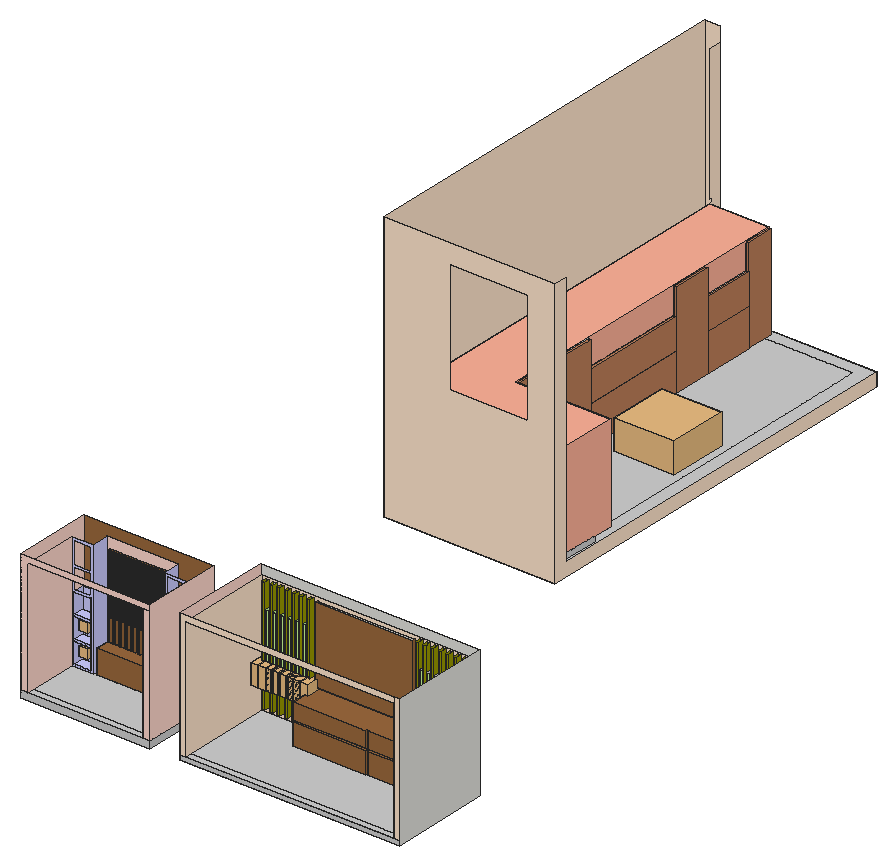
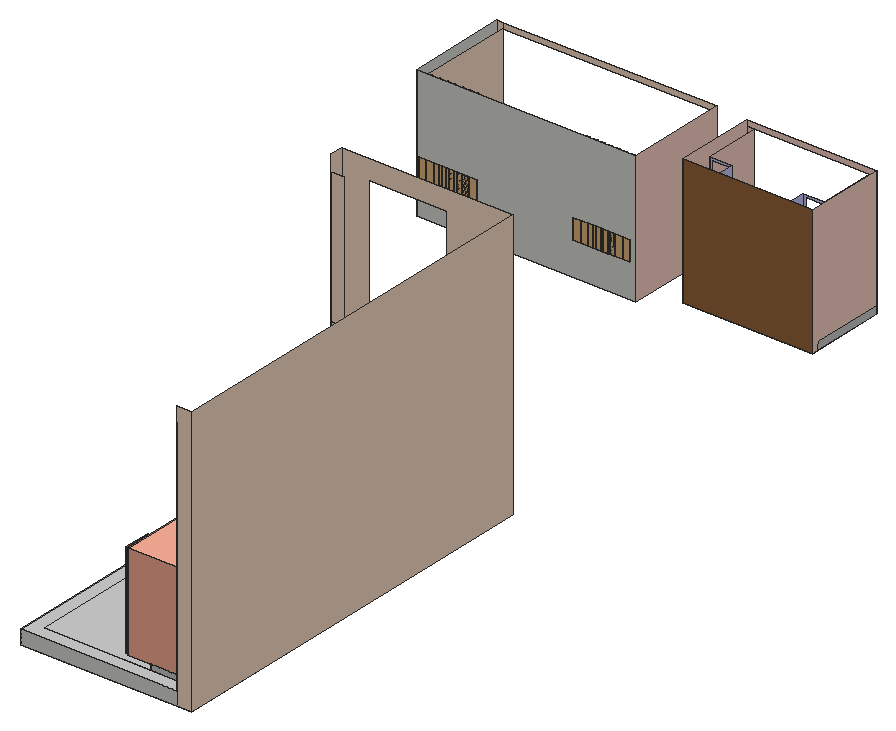
# SketchUp Ruby script. Lengths in inches.
U = 1.inch
M = Sketchup.active_model
def pt(a) = Geom::Point3d.new(a.map { |v| v * U })
def face(e, loops, mat)
  f = e.add_face(loops[0].map { |a| pt(a) })
  loops[1..].each { |l| e.add_face(l.map { |a| pt(a) }).erase! }
  f.material = f.back_material = mat if mat
  f
end
# faces: each face lists its corners as indices into pts; further lists are holes
def faces(e, pts, list, mat = nil) = list.each { |f| face(e, (f[0].is_a?(Array) ? f : [f]).map { |l| l.map { |i| pts[i] } }, mat) }
# xy, xz, yz: faces in a plane at the given z, y or x. An outline is a flat list of corners, or four numbers for a rectangle; further outlines are holes
def ring(l) = l.size == 4 ? [[l[0], l[1]], [l[2], l[1]], [l[2], l[3]], [l[0], l[3]]] : l.each_slice(2).to_a
def flat(e, list, mat, &to3) = list.each { |f| face(e, (f[0].is_a?(Array) ? f : [f]).map { |l| ring(l).map { |u, v| to3.(u, v) } }, mat) }
def xy(e, z, list, mat = nil) = flat(e, list, mat) { |x, y| [x, y, z] }
def xz(e, y, list, mat = nil) = flat(e, list, mat) { |x, z| [x, y, z] }
def yz(e, x, list, mat = nil) = flat(e, list, mat) { |y, z| [x, y, z] }
def lines(e, pts, list) = list.each { |a, b| e.add_line(pt(pts[a]), pt(pts[b])) }
# prism: a flat outline (further loops are holes) pulled along v
def prism(e, loops, v, mat = nil)
  f = face(e, loops, mat); d = Geom::Vector3d.new(v.map { |x| x * U })
  f.pushpull(f.normal.samedirection?(d) ? d.length : -d.length)
end
def box(e, o, s, mat = nil) = prism(e, [[o, [o[0] + s[0], o[1], o[2]], [o[0] + s[0], o[1] + s[1], o[2]], [o[0], o[1] + s[1], o[2]]]], [0, 0, s[2]], mat)
def at(x, y, z, deg = 0) = Geom::Transformation.translation(pt([x, y, z])) * Geom::Transformation.rotation(ORIGIN, Z_AXIS, deg.degrees)
def axes(o, x, y, z) = Geom::Transformation.new([*x, 0, *y, 0, *z, 0, *pt(o).to_a, 1])
def part(name) = M.definitions.add(name)
# library, detail: a bought-in or finely detailed component or shape, given as its bounding box
def library(name, o, s) = part(name).tap { |d| box(d.entities, o, s) }
def detail(e, o, s) = box(e.add_group.entities, o, s)
def put(e, d, t, mat = nil) = e.add_instance(d, t).tap { |i| i.material = mat if mat }
def group(e, t, mat = nil) = e.add_group.tap { |g| g.transformation = t; g.material = mat if mat }.entities
root = M.entities
M.materials.add("[Carrera Marble]").color = [207, 207, 207]
M.materials.add("[Color B01]").color = [255, 216, 204]
M.materials.add("[Color B02]").color = [255, 178, 153]
M.materials.add("[Color C01]").color = [255, 229, 204]
M.materials.add("[Color E07]").color = [153, 153, 0]
M.materials.add("[Color F02]").color = [204, 255, 153]
M.materials.add("[Color I01]").color = [204, 204, 255]
M.materials.add("[Wood Floor]").color = [155, 105, 61]
M.materials.add("[Wood Veneer 02]").color = [190, 128, 91]
c1 = library("Dome Light",[-12,-12,0],[24,24,12])
c2 = library("Spot Light\#1",[-5.1,-5.1,-11.05],[10.2,10.2,11.05])
c3 = library("Spot Light\#2",[-5.1,-5.1,-11.05],[10.2,10.2,11.05])
c4 = library("Omni Light",[-12,-12,-12],[24,24,24])
prism(root,[[[126.97,824.11,13.18],[126.78,870.57,13.18],[130.77,870.59,13.18],[130.95,824.12,13.18]]],[0,0,114.09],"[Wood Veneer 02]")
prism(root,[[[126.97,933.65,13.18],[126.59,966.6875,13.18],[130.19,966.73,13.18],[130.56,933.6875,13.18]]],[0,0,114.09],"[Wood Veneer 02]")
xy(root,-10.3125,[[38.18,499.97,244.12,983.1]])
xy(root,0,[[0,0,156.26,96.1875],[190.88,1.64,455.07,122.89]])
xy(root,5.5,[[197.89,1.64,448.06,8.66],[197.89,8.66,448.06,8.66,448.06,115.88,386.51,115.88,386.51,80.51,353.55,80.51,353.55,82.13,351.17,82.13,351.17,80.51,263.76,80.51,263.76,115.88,197.89,115.88]],"[Carrera Marble]")
xy(root,6.0625,[[228.71,515.38,244.12,515.38,244.12,983.1,55.53,983.1,55.53,967.6875,228.71,967.6875],[99.17,515.38,228.71,967.6875]],"[Carrera Marble]")
xy(root,8.6875,[[39.83,68.2,44.81,87.7],[47.15,68.2,52.13,84.32],[54.47,68.2,59.45,84.32],[61.79,68.2,66.77,84.32],[69.11,68.2,74.1,84.32],
  [76.43,68.2,81.42,84.32],[83.76,68.2,88.74,87.7],[91.08,68.2,96.06,84.32],[98.4,68.2,103.38,84.32],[105.72,68.2,110.7,87.7],
  [113.04,68.2,116.32,84.32],[47.15,84.32,52.13,87.7],[54.47,84.32,59.45,87.7],[61.79,84.32,66.77,87.7],[69.11,84.32,74.1,87.7],
  [76.43,84.32,81.42,87.7],[91.08,84.32,96.06,87.7],[98.4,84.32,103.38,87.7]])
xy(root,8.6875,[[8.49,0,147.15,8.49],[8.49,8.49,147.15,8.49,147.15,67.26,120.02,67.26,120.02,87.7,113.04,87.7,113.04,84.32,116.32,84.32,116.32,68.2,37.49,68.2,37.49,87.7,34.3,87.7,34.3,67.26,8.49,67.26]],"[Carrera Marble]")
xy(root,11.37,[[11.17,67.26,31.62,80.32]],"[Color I01]")
xy(root,11.4,[[122.73,67.26,144.4375,90.2]],"[Color I01]")
xy(root,11.5,[[202.89,109.94,206.54,115.88],[211.9,109.94,215.55,115.88],[215.55,109.94,215.57,115.88],[220.91,109.94,224.56,115.88],[229.92,109.94,233.57,115.88],
  [238.94,109.94,242.58,115.88],[247.95,109.94,251.59,115.88],[256.96,109.94,260.6,115.88],[388.06,109.94,391.7,115.88],[397.22,109.94,400.87,115.88],
  [406.39,109.94,410.03,115.88],[415.56,109.94,419.2,115.88],[419.2,109.94,419.22,115.88],[424.72,109.94,428.37,115.88],[433.89,109.94,437.53,115.88],
  [443.06,109.94,446.7,115.88]])
xy(root,12.375,[[55.53,515.38,55.53,967.6875,126.78,967.6875,126.78,823.17,131.14,823.17,131.14,696.23,126.78,696.23,126.78,586.56,241.2,586.56,241.2,515.38]])
xy(root,13.18,[[129.68,586.56,164.24,588.31],[164.74,586.56,240.3,588.31],[126.97,589.61,126.78,649.43,130.09,649.44,130.28,589.62],[126.97,650.36,126.78,695.33,130.09,695.35,130.28,650.375],[126.78,871.47,130.59,932.72]])
xy(root,31.1875,[[263.76,80.51,351.17,80.51,351.17,82.13,353.55,82.13,353.55,80.51,386.51,80.51,386.51,84.57,263.76,84.57]],"[Wood Floor]")
xy(root,33.9375,[[263.76,80.51,263.76,84.57,386.51,84.57,386.51,80.51,353.55,80.51,353.55,82.13,351.17,82.13,351.17,80.51]],"[Wood Floor]")
xy(root,36.07,[[11.17,67.26,31.62,80.32]],"[Color I01]")
xy(root,36.09,[[122.73,67.26,144.4375,90.2]])
xy(root,37.16,[[37.49,68.2,116.32,84.32]],"[Wood Floor]")
xy(root,38.07,[[11.17,67.26,31.62,80.32]],"[Color I01]")
xy(root,38.09,[[122.73,67.26,144.4375,90.2]],"[Color I01]")
xy(root,52.9375,[[263.76,80.51,351.17,80.51,351.17,82.13,353.55,82.13,353.55,80.51,386.51,80.51,386.51,115.88,263.76,115.88]],"[Wood Floor]")
xy(root,56.35,[[264.93,112.26,382.43,115.88]],"[Wood Floor]")
xy(root,58.06,[[126.78,696.23,131.14,823.17],[126.78,871.47,130.59,932.72]],"[Wood Veneer 02]")
xy(root,58.66,[[126.78,696.23,131.14,823.17],[115.09,871.47,126.28,932.72],[126.28,871.47,126.78,932.72],[126.78,871.47,130.59,932.72]])
xy(root,59.39,[[410.97,109.94,414.62,115.88]])
xy(root,59.66,[[243.44,109.94,247.09,115.88],[252.45,109.94,256.1,115.88],[392.64,109.94,396.28,115.88],[401.81,109.94,405.45,115.88]])
xy(root,60,[[420.14,109.94,423.78,115.88],[429.31,109.94,432.95,115.88]])
xy(root,60.5,[[207.4,109.94,211.04,115.88],[216.41,109.94,220.05,115.88],[225.42,109.94,229.06,115.88],[234.43,109.94,238.08,115.88]])
xy(root,60.52,[[438.47,109.94,442.12,115.88]])
xy(root,62.77,[[11.17,67.26,31.62,80.32]],"[Color I01]")
xy(root,62.78,[[122.73,67.26,144.4375,90.2]])
xy(root,64.25,[[41.15,84.32,43.49,87.7],[48.47,84.32,50.81,87.7],[55.79,84.32,58.13,87.7],[63.11,84.32,65.45,87.7],[70.43,84.32,72.77,87.7],
  [77.76,84.32,80.1,87.7],[85.08,84.32,87.42,87.7],[92.4,84.32,94.74,87.7],[99.72,84.32,102.06,87.7],[107.04,84.32,109.38,87.7],
  [114.36,84.32,116.7,87.7]])
xy(root,64.77,[[11.17,67.26,31.62,80.32]],"[Color I01]")
xy(root,64.78,[[122.73,67.26,144.4375,90.2]],"[Color I01]")
xy(root,80.6,[[164.74,586.56,240.3,588.31]],"[Wood Veneer 02]")
xy(root,95.53,[[115.09,871.47,126.28,932.72],[126.28,871.47,126.78,932.72]])
xy(root,95.53,[[126.78,696.23,131.14,823.17],[126.78,871.47,130.59,932.72]],"[Wood Veneer 02]")
xy(root,127.26,[[129.68,586.56,164.24,588.31],[126.97,589.61,130.28,589.62,130.09,649.44,126.78,649.43],[126.97,650.36,130.28,650.375,130.09,695.35,126.78,695.33]],"[Wood Veneer 02]")
xz(root,0,[[0,0,156.26,8.6875]],"[Carrera Marble]")
xz(root,0,[[0,8.6875,8.49,8.6875,8.49,148.5,156.26,148.5,156.26,155.125,0,155.125],[147.15,8.6875,156.26,148.5]],"[Color B01]")
xz(root,1.64,[[190.88,0,455.07,5.5]],"[Carrera Marble]")
xz(root,1.64,[[190.88,5.5,197.89,5.5,197.89,151.1875,448.06,151.1875,448.06,158,190.88,158],[448.06,5.5,455.07,158]],"[Color C01]")
xz(root,67.26,[[[8.49,8.6875,34.3,147.5625],[11.17,118.18,31.62,144.88],[11.17,64.77,31.62,89.48],[11.17,11.37,31.62,36.07],[11.17,38.07,31.62,62.77],[11.17,91.48,31.62,116.18]],[[120.02,8.6875,147.15,147.5625],[122.73,118.16,144.4375,144.85],[122.73,64.78,144.4375,89.47],[122.73,38.09,144.4375,62.78],[122.73,11.4,144.4375,36.09],[122.73,91.47,144.4375,116.16]]],"[Color I01]")
xz(root,68.2,[[37.49,8.6875,116.32,37.16]],"[Wood Floor]")
xz(root,80.32,[[11.17,11.37,31.62,36.07],[11.17,38.07,31.62,62.77],[11.17,64.77,31.62,89.48]],"[Color I01]")
xz(root,80.51,[[263.76,5.5,351.17,31.1875],[353.55,5.5,386.51,31.1875],[263.76,33.9375,351.17,52.9375],[353.55,33.9375,386.51,52.9375]],"[Wood Floor]")
xz(root,82.13,[[351.17,5.5,353.55,31.1875],[351.17,33.9375,353.55,52.9375]],"[Wood Floor]")
xz(root,84.32,[[37.49,8.6875,52.13,37.16],[52.13,8.6875,59.45,37.16],[59.45,8.6875,66.77,37.16],[66.77,8.6875,74.1,37.16],[74.1,8.6875,81.42,37.16],
  [81.42,8.6875,96.06,37.16],[96.06,8.6875,103.38,37.16],[103.38,8.6875,110.7,37.16],[110.7,8.6875,116.32,37.16]])
xz(root,84.57,[[263.76,31.1875,386.51,33.9375]],"[Wood Floor]")
xz(root,87.7,[[[34.3,8.6875,37.49,8.6875,37.49,135.5625,39.83,135.5625,39.83,8.6875,44.81,8.6875,44.81,135.5625,47.15,135.5625,47.15,8.6875,52.13,8.6875,52.13,135.5625,54.47,135.5625,54.47,8.6875,59.45,8.6875,59.45,135.5625,61.79,135.5625,61.79,8.6875,66.77,8.6875,66.77,135.5625,69.11,135.5625,69.11,8.6875,74.1,8.6875,74.1,135.5625,76.43,135.5625,76.43,8.6875,81.42,8.6875,81.42,135.5625,83.76,135.5625,83.76,8.6875,88.74,8.6875,88.74,135.5625,91.08,135.5625,91.08,8.6875,96.06,8.6875,96.06,135.5625,98.4,135.5625,98.4,8.6875,103.38,8.6875,103.38,135.5625,105.72,135.5625,105.72,8.6875,110.7,8.6875,110.7,135.5625,113.04,135.5625,113.04,8.6875,120.02,8.6875,120.02,148.5,34.3,148.5],[41.15,64.25,43.49,135.5625],[48.47,64.25,50.81,135.5625],[55.79,64.25,58.13,135.5625],[63.11,64.25,65.45,135.5625],[70.43,64.25,72.77,135.5625],[77.76,64.25,80.1,135.5625],[85.08,64.25,87.42,135.5625],[92.4,64.25,94.74,135.5625],[99.72,64.25,102.06,135.5625],[107.04,64.25,109.38,135.5625],[114.36,64.25,116.7,135.5625]]],"[Color B01]")
xz(root,90.2,[[122.73,11.4,144.4375,36.09],[122.73,38.09,144.4375,62.78],[122.73,64.78,144.4375,89.47]],"[Color I01]")
xz(root,96.1875,[[0,0,156.26,155.125]],"[Wood Floor]")
xz(root,109.94,[[202.89,11.5,206.54,149],[211.9,11.5,215.55,149],[220.91,11.5,224.56,149],[229.92,11.5,233.57,149],[238.94,11.5,242.58,149],
  [247.95,11.5,251.59,149],[256.96,11.5,260.6,149],[388.06,11.5,391.7,149],[397.22,11.5,400.87,149],[406.39,11.5,410.03,149],
  [415.56,11.5,419.2,149],[424.72,11.5,428.37,149],[433.89,11.5,437.53,149],[443.06,11.5,446.7,149]],"[Color E07]")
xz(root,109.94,[[410.97,59.39,414.62,120.1875],[243.44,59.66,247.09,120.1875],[252.45,59.66,256.1,120.1875],[392.64,59.66,396.28,120.1875],[401.81,59.66,405.45,120.1875],
  [420.14,60,423.78,120.1875],[429.31,60,432.95,120.1875],[207.4,60.5,211.04,120.1875],[216.41,60.5,220.05,120.1875],[225.42,60.5,229.06,120.1875],
  [234.43,60.5,238.08,120.1875],[438.47,60.52,442.12,120.1875]],"[Color F02]")
xz(root,112.26,[[264.93,56.35,382.43,147.04]],"[Wood Floor]")
xz(root,115.88,[[211.9,11.5,215.55,149],[220.91,11.5,224.56,149],[229.92,11.5,233.57,149],[238.94,11.5,242.58,149],[247.95,11.5,251.59,149],
  [256.96,11.5,260.6,149],[388.06,11.5,391.7,149],[397.22,11.5,400.87,149],[406.39,11.5,410.03,149],[415.56,11.5,419.2,149],
  [424.72,11.5,428.37,149],[433.89,11.5,437.53,149],[443.06,11.5,446.7,149],[410.97,59.39,414.62,120.1875],[243.44,59.66,247.09,120.1875],
  [252.45,59.66,256.1,120.1875],[392.64,59.66,396.28,120.1875],[401.81,59.66,405.45,120.1875],[420.14,60,423.78,120.1875],[429.31,60,432.95,120.1875],
  [207.4,60.5,211.04,120.1875],[216.41,60.5,220.05,120.1875],[225.42,60.5,229.06,120.1875],[234.43,60.5,238.08,120.1875],[438.47,60.52,442.12,120.1875]])
xz(root,115.88,[[[197.89,5.5,263.76,5.5,263.76,52.9375,386.51,52.9375,386.51,5.5,448.06,5.5,448.06,151.1875,197.89,151.1875],[264.93,56.35,382.43,147.04],[202.89,11.5,206.54,149],[211.9,11.5,215.55,149],[220.91,11.5,224.56,149],[229.92,11.5,233.57,149],[238.94,11.5,242.58,149],[247.95,11.5,251.59,149],[256.96,11.5,260.6,149],[388.06,11.5,391.7,149],[397.22,11.5,400.87,149],[406.39,11.5,410.03,149],[415.56,11.5,419.2,149],[424.72,11.5,428.37,149],[433.89,11.5,437.53,149],[443.06,11.5,446.7,149],[410.97,59.39,414.62,120.1875],[243.44,59.66,247.09,120.1875],[252.45,59.66,256.1,120.1875],[401.81,59.66,405.45,120.1875],[392.64,59.66,396.28,120.1875],[420.14,60,423.78,120.1875],[429.31,60,432.95,120.1875],[207.4,60.5,211.04,120.1875],[216.41,60.5,220.05,120.1875],[225.42,60.5,229.06,120.1875],[234.43,60.5,238.08,120.1875],[438.47,60.52,442.12,120.1875]]],"[Color C01]")
xz(root,122.89,[[190.88,0,455.07,158]])
xz(root,499.97,[[[38.18,-10.3125,244.12,313],[116.72,153.625,211.22,289.75]]],"[Color C01]")
xz(root,515.38,[[99.17,6.0625,228.71,12.375],[55.53,12.375,99.17,132.5625],[99.17,12.375,228.71,132.5625],[228.71,12.375,228.71,132.5625,243.82,132.5625,243.82,128.0625,241.2,128.0625,241.2,12.375]])
xz(root,515.38,[[228.71,6.0625,228.71,12.375,241.2,12.375,241.2,128.0625,243.82,128.0625,243.82,132.5625,228.71,132.5625,228.71,294.5,244.12,294.5,244.12,6.0625]],"[Color C01]")
xz(root,586.56,[[129.68,13.18,164.24,127.26],[164.74,13.18,240.3,80.6]])
xz(root,588.31,[[129.68,13.18,164.24,127.26],[164.74,13.18,240.3,80.6]],"[Wood Veneer 02]")
xz(root,696.23,[[126.78,12.375,131.14,58.06],[126.78,58.66,131.14,95.53]],"[Wood Veneer 02]")
xz(root,823.17,[[126.78,12.375,131.14,58.06],[126.78,58.66,131.14,95.53]],"[Color B02]")
xz(root,871.47,[[115.09,58.66,126.28,95.53],[126.28,58.66,126.78,95.53]])
xz(root,871.47,[[126.78,13.18,130.59,58.06],[126.78,58.66,130.59,95.53]],"[Wood Veneer 02]")
xz(root,932.72,[[115.09,58.66,126.28,95.53],[126.28,58.66,126.78,95.53]])
xz(root,932.72,[[126.78,13.18,130.59,58.06]],"[Color B02]")
xz(root,932.72,[[126.78,58.66,130.59,95.53]],"[Wood Veneer 02]")
xz(root,983.1,[[55.53,-10.3125,244.12,6.0625]])
xz(root,983.1,[[38.18,-10.3125,55.53,313]],"[Color C01]")
yz(root,0,[[0,0,87.7,8.6875]],"[Carrera Marble]")
yz(root,0,[[87.7,0,87.7,8.6875,0,8.6875,0,155.125,96.1875,155.125,96.1875,0]],"[Color B01]")
yz(root,8.49,[[0,8.6875,67.26,147.5625]],"[Color B01]")
yz(root,11.17,[[67.26,11.37,80.32,36.07],[67.26,38.07,80.32,62.77],[67.26,64.77,80.32,89.48]],"[Color I01]")
yz(root,31.62,[[67.26,36.07,80.32,38.07],[67.26,62.77,80.32,64.77]])
yz(root,31.62,[[67.26,11.37,80.32,36.07],[67.26,38.07,80.32,62.77],[67.26,64.77,80.32,89.48]],"[Color I01]")
yz(root,34.3,[[67.26,8.6875,87.7,147.5625]],"[Color I01]")
yz(root,37.49,[[68.2,8.6875,84.32,37.16]],"[Wood Floor]")
yz(root,38.18,[[499.97,-10.3125,983.1,313]],"[Color C01]")
yz(root,48.47,[[84.32,64.25,87.7,135.5625]],"[Wood Floor]")
yz(root,52.13,[[84.32,8.6875,87.7,135.5625]],"[Wood Floor]")
yz(root,55.53,[[515.38,12.375,967.6875,128.0625]])
yz(root,55.53,[[967.6875,6.0625,983.1,6.0625,983.1,294.5,967.6875,294.5,967.6875,132.5625,971,132.5625,971,128.0625,967.6875,128.0625]],"[Color C01]")
yz(root,55.79,[[84.32,64.25,87.7,135.5625]],"[Wood Floor]")
yz(root,59.45,[[84.32,8.6875,87.7,135.5625]],"[Wood Floor]")
yz(root,63.11,[[84.32,64.25,87.7,135.5625]],"[Wood Floor]")
yz(root,66.77,[[84.32,8.6875,87.7,135.5625]],"[Wood Floor]")
yz(root,70.43,[[84.32,64.25,87.7,135.5625]],"[Wood Floor]")
yz(root,74.1,[[84.32,8.6875,87.7,135.5625]],"[Wood Floor]")
yz(root,77.76,[[84.32,64.25,87.7,135.5625]],"[Wood Floor]")
yz(root,81.42,[[84.32,8.6875,87.7,135.5625]],"[Wood Floor]")
yz(root,85.08,[[84.32,64.25,87.7,135.5625]],"[Wood Floor]")
yz(root,92.4,[[84.32,64.25,87.7,135.5625]],"[Wood Floor]")
yz(root,96.06,[[84.32,8.6875,87.7,135.5625]],"[Wood Floor]")
yz(root,99.72,[[84.32,64.25,87.7,135.5625]],"[Wood Floor]")
yz(root,103.38,[[84.32,8.6875,87.7,135.5625]],"[Wood Floor]")
yz(root,107.04,[[84.32,64.25,87.7,135.5625]],"[Wood Floor]")
yz(root,110.7,[[84.32,8.6875,87.7,135.5625]],"[Wood Floor]")
yz(root,114.36,[[84.32,64.25,87.7,135.5625]],"[Wood Floor]")
yz(root,115.09,[[871.47,58.66,932.72,95.53]])
yz(root,116.32,[[68.2,8.6875,84.32,37.16]],"[Wood Floor]")
yz(root,120.02,[[67.26,8.6875,87.7,147.5625]],"[Color I01]")
yz(root,122.73,[[67.26,11.4,90.2,36.09],[67.26,38.09,90.2,62.78],[67.26,64.78,90.2,89.47]],"[Color I01]")
yz(root,126.28,[[871.47,58.66,932.72,95.53]])
yz(root,126.78,[[871.47,13.18,932.72,58.06],[696.23,58.66,823.17,95.53],[871.47,58.66,932.72,95.53]])
yz(root,129.68,[[586.56,13.18,588.31,127.26]])
yz(root,130.59,[[871.47,13.18,932.72,58.06],[871.47,58.66,932.72,95.53]],"[Wood Veneer 02]")
yz(root,131.14,[[696.23,12.375,823.17,58.06],[696.23,58.66,823.17,95.53]],"[Wood Veneer 02]")
yz(root,144.4375,[[67.26,36.09,90.2,38.09],[67.26,62.78,90.2,64.78]])
yz(root,144.4375,[[67.26,11.4,90.2,36.09],[67.26,38.09,90.2,62.78],[67.26,64.78,90.2,89.47]],"[Color I01]")
yz(root,147.15,[[0,8.6875,67.26,147.5625]],"[Color B01]")
yz(root,156.26,[[0,0,87.7,8.6875]],"[Carrera Marble]")
yz(root,156.26,[[87.7,0,96.1875,0,96.1875,155.125,0,155.125,0,8.6875,87.7,8.6875]],"[Color B01]")
yz(root,164.24,[[586.56,13.18,588.31,127.26]],"[Color B02]")
yz(root,164.74,[[586.56,13.18,588.31,80.6]])
yz(root,190.88,[[1.64,0,122.89,158]],"[Color B01]")
yz(root,197.89,[[1.64,5.5,115.88,151.1875]],"[Color C01]")
yz(root,202.89,[[109.94,11.5,115.88,149]],"[Color E07]")
yz(root,206.54,[[109.94,11.5,115.88,149]],"[Color E07]")
yz(root,207.4,[[109.94,60.5,115.88,120.1875]],"[Color F02]")
yz(root,211.04,[[109.94,60.5,115.88,120.1875]],"[Color F02]")
yz(root,211.9,[[109.94,11.5,115.88,149]],"[Color E07]")
yz(root,215.55,[[109.94,11.5,115.88,149]],"[Color E07]")
yz(root,216.41,[[109.94,60.5,115.88,120.1875]],"[Color F02]")
yz(root,220.05,[[109.94,60.5,115.88,120.1875]],"[Color F02]")
yz(root,220.91,[[109.94,11.5,115.88,149]],"[Color E07]")
yz(root,224.56,[[109.94,11.5,115.88,149]],"[Color E07]")
yz(root,225.42,[[109.94,60.5,115.88,120.1875]],"[Color F02]")
yz(root,229.06,[[109.94,60.5,115.88,120.1875]],"[Color F02]")
yz(root,229.92,[[109.94,11.5,115.88,149]],"[Color E07]")
yz(root,233.57,[[109.94,11.5,115.88,149]],"[Color E07]")
yz(root,234.43,[[109.94,60.5,115.88,120.1875]],"[Color F02]")
yz(root,238.08,[[109.94,60.5,115.88,120.1875]],"[Color F02]")
yz(root,238.94,[[109.94,11.5,115.88,149]],"[Color E07]")
yz(root,240.3,[[586.56,13.18,588.31,80.6]],"[Wood Veneer 02]")
yz(root,242.58,[[109.94,11.5,115.88,149]],"[Color E07]")
yz(root,243.44,[[109.94,59.66,115.88,120.1875]],"[Color F02]")
yz(root,244.12,[[499.97,-10.3125,983.1,-10.3125,983.1,6.0625,515.38,6.0625,515.38,313,499.97,313]],"[Color C01]")
yz(root,247.09,[[109.94,59.66,115.88,120.1875]])
yz(root,247.95,[[109.94,11.5,115.88,149]],"[Color E07]")
yz(root,251.59,[[109.94,11.5,115.88,149]],"[Color E07]")
yz(root,252.45,[[109.94,59.66,115.88,120.1875]],"[Color F02]")
yz(root,256.1,[[109.94,59.66,115.88,120.1875]],"[Color F02]")
yz(root,256.96,[[109.94,11.5,115.88,149]],"[Color E07]")
yz(root,260.6,[[109.94,11.5,115.88,149]],"[Color E07]")
yz(root,263.76,[[80.51,5.5,80.51,31.1875,84.57,31.1875,84.57,33.9375,80.51,33.9375,80.51,52.9375,115.88,52.9375,115.88,5.5]],"[Wood Floor]")
yz(root,264.93,[[112.26,56.35,115.88,147.04]],"[Wood Floor]")
yz(root,351.17,[[80.51,5.5,82.13,31.1875],[80.51,33.9375,82.13,52.9375]],"[Wood Floor]")
yz(root,353.55,[[80.51,5.5,82.13,31.1875],[80.51,33.9375,82.13,52.9375]],"[Wood Floor]")
yz(root,382.43,[[112.26,56.35,115.88,147.04]],"[Wood Floor]")
yz(root,386.51,[[80.51,5.5,115.88,5.5,115.88,52.9375,80.51,52.9375,80.51,33.9375,84.57,33.9375,84.57,31.1875,80.51,31.1875]],"[Wood Floor]")
yz(root,388.06,[[109.94,11.5,115.88,149]],"[Color E07]")
yz(root,391.7,[[109.94,11.5,115.88,149]],"[Color E07]")
yz(root,392.64,[[109.94,59.66,115.88,120.1875]])
yz(root,396.28,[[109.94,59.66,115.88,120.1875]],"[Color F02]")
yz(root,397.22,[[109.94,11.5,115.88,149]],"[Color E07]")
yz(root,400.87,[[109.94,11.5,115.88,149]],"[Color E07]")
yz(root,401.81,[[109.94,59.66,115.88,120.1875]])
yz(root,405.45,[[109.94,59.66,115.88,120.1875]],"[Color F02]")
yz(root,406.39,[[109.94,11.5,115.88,149]],"[Color E07]")
yz(root,410.03,[[109.94,11.5,115.88,149]],"[Color E07]")
yz(root,410.97,[[109.94,59.39,115.88,120.1875]])
yz(root,414.62,[[109.94,59.39,115.88,120.1875]],"[Color F02]")
yz(root,415.56,[[109.94,11.5,115.88,149]],"[Color E07]")
yz(root,419.2,[[109.94,11.5,115.88,149]],"[Color E07]")
yz(root,420.14,[[109.94,60,115.88,120.1875]])
yz(root,423.78,[[109.94,60,115.88,120.1875]],"[Color F02]")
yz(root,424.72,[[109.94,11.5,115.88,149]],"[Color E07]")
yz(root,428.37,[[109.94,11.5,115.88,149]],"[Color E07]")
yz(root,429.31,[[109.94,60,115.88,120.1875]])
yz(root,432.95,[[109.94,60,115.88,120.1875]],"[Color F02]")
yz(root,433.89,[[109.94,11.5,115.88,149]],"[Color E07]")
yz(root,437.53,[[109.94,11.5,115.88,149]],"[Color E07]")
yz(root,438.47,[[109.94,60.52,115.88,120.1875]])
yz(root,442.12,[[109.94,60.52,115.88,120.1875]],"[Color F02]")
yz(root,443.06,[[109.94,11.5,115.88,149]],"[Color E07]")
yz(root,446.7,[[109.94,11.5,115.88,149]],"[Color E07]")
yz(root,448.06,[[1.64,5.5,115.88,151.1875]],"[Color C01]")
yz(root,455.07,[[1.64,0,122.89,158]])
p = [[126.97,589.61,13.18],[126.97,589.61,127.26],[126.78,649.43,127.26],[126.78,649.43,13.18],[130.28,589.62,13.18],[130.28,589.62,127.26],
  [130.09,649.44,13.18],[130.09,649.44,127.26],[126.78,695.33,127.26],[126.78,695.33,13.18],[126.97,650.36,13.18],[126.97,650.36,127.26],
  [130.28,650.375,13.18],[130.28,650.375,127.26],[130.09,695.35,13.18],[130.09,695.35,127.26]]
faces(root,p,[[0,1,2,3],[1,0,4,5],[8,9,10,11]])
faces(root,p,[[5,4,6,7],[3,2,7,6],[11,10,12,13],[14,15,13,12]],"[Wood Veneer 02]")
faces(root,p,[[9,8,15,14]],"[Color B02]")
put(root,c1,axes([182.73,745.84,6.0625],[3,0,0],[0,3,0],[0,0,3]),"[Color I01]")
g1 = group(root,at(55.53,515.38,6.0625),"[Carrera Marble]")
xy(g1,0,[[43.64,0,185.67,48.25]])
xy(g1,6.3125,[[0,0,185.67,0,185.67,48.25,43.64,48.25,43.64,452.31,0,452.31]],"[Carrera Marble]")
xz(g1,0,[[43.64,0,185.67,6.3125]])
xz(g1,48.25,[[43.64,0,185.67,6.3125]],"[Carrera Marble]")
xz(g1,452.31,[[0,0,43.64,6.3125]])
yz(g1,43.64,[[48.25,0,452.31,6.3125]])
yz(g1,185.67,[[0,0,48.25,6.3125]],"[Carrera Marble]")
g2 = group(root,at(37.49,84.32,8.6875),"[Wood Floor]")
xy(g2,126.875,[[0,0,2.34,3.375],[3.66,0,6,3.375],[7.32,0,9.66,3.375],[10.98,0,13.32,3.375],[14.64,0,16.98,3.375],
  [18.3,0,20.64,3.375],[21.96,0,24.3,3.375],[25.625,0,27.96,3.375],[29.29,0,31.625,3.375],[32.95,0,35.29,3.375],
  [36.61,0,38.95,3.375],[40.27,0,42.61,3.375],[43.93,0,46.27,3.375],[47.59,0,49.93,3.375],[51.25,0,53.59,3.375],
  [54.91,0,57.25,3.375],[58.57,0,60.91,3.375],[62.23,0,64.57,3.375],[65.89,0,68.23,3.375],[69.55,0,71.89,3.375],
  [73.21,0,75.55,3.375],[76.875,0,79.21,3.375]],"[Wood Floor]")
xz(g2,0,[[0,0,2.34,126.875],[7.32,0,9.66,126.875],[14.64,0,16.98,126.875],[21.96,0,24.3,126.875],[29.29,0,31.625,126.875],
  [36.61,0,38.95,126.875],[43.93,0,46.27,126.875],[51.25,0,53.59,126.875],[58.57,0,60.91,126.875],[65.89,0,68.23,126.875],
  [73.21,0,75.55,126.875],[3.66,55.5625,6,126.875],[10.98,55.5625,13.32,126.875],[18.3,55.5625,20.64,126.875],[25.625,55.5625,27.96,126.875],
  [32.95,55.5625,35.29,126.875],[40.27,55.5625,42.61,126.875],[47.59,55.5625,49.93,126.875],[54.91,55.5625,57.25,126.875],[62.23,55.5625,64.57,126.875],
  [69.55,55.5625,71.89,126.875],[76.875,55.5625,79.21,126.875]],"[Wood Floor]")
yz(g2,0,[[0,0,3.375,126.875]],"[Wood Floor]")
yz(g2,2.34,[[0,0,3.375,126.875]],"[Wood Floor]")
yz(g2,3.66,[[0,55.5625,3.375,126.875]],"[Wood Floor]")
yz(g2,6,[[0,55.5625,3.375,126.875]],"[Wood Floor]")
yz(g2,7.32,[[0,0,3.375,126.875]],"[Wood Floor]")
yz(g2,9.66,[[0,0,3.375,126.875]],"[Wood Floor]")
yz(g2,13.32,[[0,55.5625,3.375,126.875]])
yz(g2,16.98,[[0,0,3.375,126.875]],"[Wood Floor]")
yz(g2,20.64,[[0,55.5625,3.375,126.875]],"[Wood Floor]")
yz(g2,24.3,[[0,0,3.375,126.875]],"[Wood Floor]")
yz(g2,27.96,[[0,55.5625,3.375,126.875]],"[Wood Floor]")
yz(g2,31.625,[[0,0,3.375,126.875]],"[Wood Floor]")
yz(g2,35.29,[[0,55.5625,3.375,126.875]],"[Wood Floor]")
yz(g2,38.95,[[0,0,3.375,126.875]],"[Wood Floor]")
yz(g2,42.61,[[0,55.5625,3.375,126.875]],"[Wood Floor]")
yz(g2,46.27,[[0,0,3.375,126.875]],"[Wood Floor]")
yz(g2,49.93,[[0,55.5625,3.375,126.875]],"[Wood Floor]")
yz(g2,51.25,[[0,0,3.375,126.875]])
yz(g2,53.59,[[0,0,3.375,126.875]],"[Wood Floor]")
yz(g2,57.25,[[0,55.5625,3.375,126.875]],"[Wood Floor]")
yz(g2,60.91,[[0,0,3.375,126.875]],"[Wood Floor]")
yz(g2,64.57,[[0,55.5625,3.375,126.875]],"[Wood Floor]")
yz(g2,68.23,[[0,0,3.375,126.875]],"[Wood Floor]")
yz(g2,71.89,[[0,55.5625,3.375,126.875]],"[Wood Floor]")
yz(g2,75.55,[[0,0,3.375,126.875]],"[Wood Floor]")
yz(g2,79.21,[[0,55.5625,3.375,126.875]],"[Wood Floor]")
g3 = group(root,at(55.53,515.38,12.375),"[Color B02]")
xy(g3,115.6875,[[0,0,185.67,0,185.67,71.18,71.25,71.18,71.25,452.31,0,452.31]])
xz(g3,71.18,[[71.25,0,185.67,115.6875]])
xz(g3,452.31,[[0,0,71.25,115.6875]],"[Color B02]")
yz(g3,71.25,[[71.18,0,452.31,115.6875]],"[Color B02]")
yz(g3,185.67,[[0,0,71.18,115.6875]],"[Color B02]")
put(root,c2,at(22.06,72.69,32.55))
put(root,c3,at(131.8,77.15,33.53))
put(root,c4,at(254.85,110.91,52.64))
put(root,c4,at(245.6,110.91,52.64))
put(root,c4,at(236.79,110.91,52.64))
put(root,c4,at(227.97,110.91,52.64))
put(root,c4,at(218.91,110.91,52.64))
put(root,c4,at(210.22,110.91,52.64))
put(root,c4,at(394.85,110.91,52.64))
put(root,c4,at(403.97,110.91,52.64))
put(root,c4,at(413.22,110.91,52.64))
put(root,c4,at(422.41,110.91,52.64))
put(root,c4,at(431.79,110.91,52.64))
put(root,c4,at(440.97,110.91,52.64))
put(root,c2,at(22.06,72.69,60.55))
put(root,c3,at(131.8,77.15,61.47))
